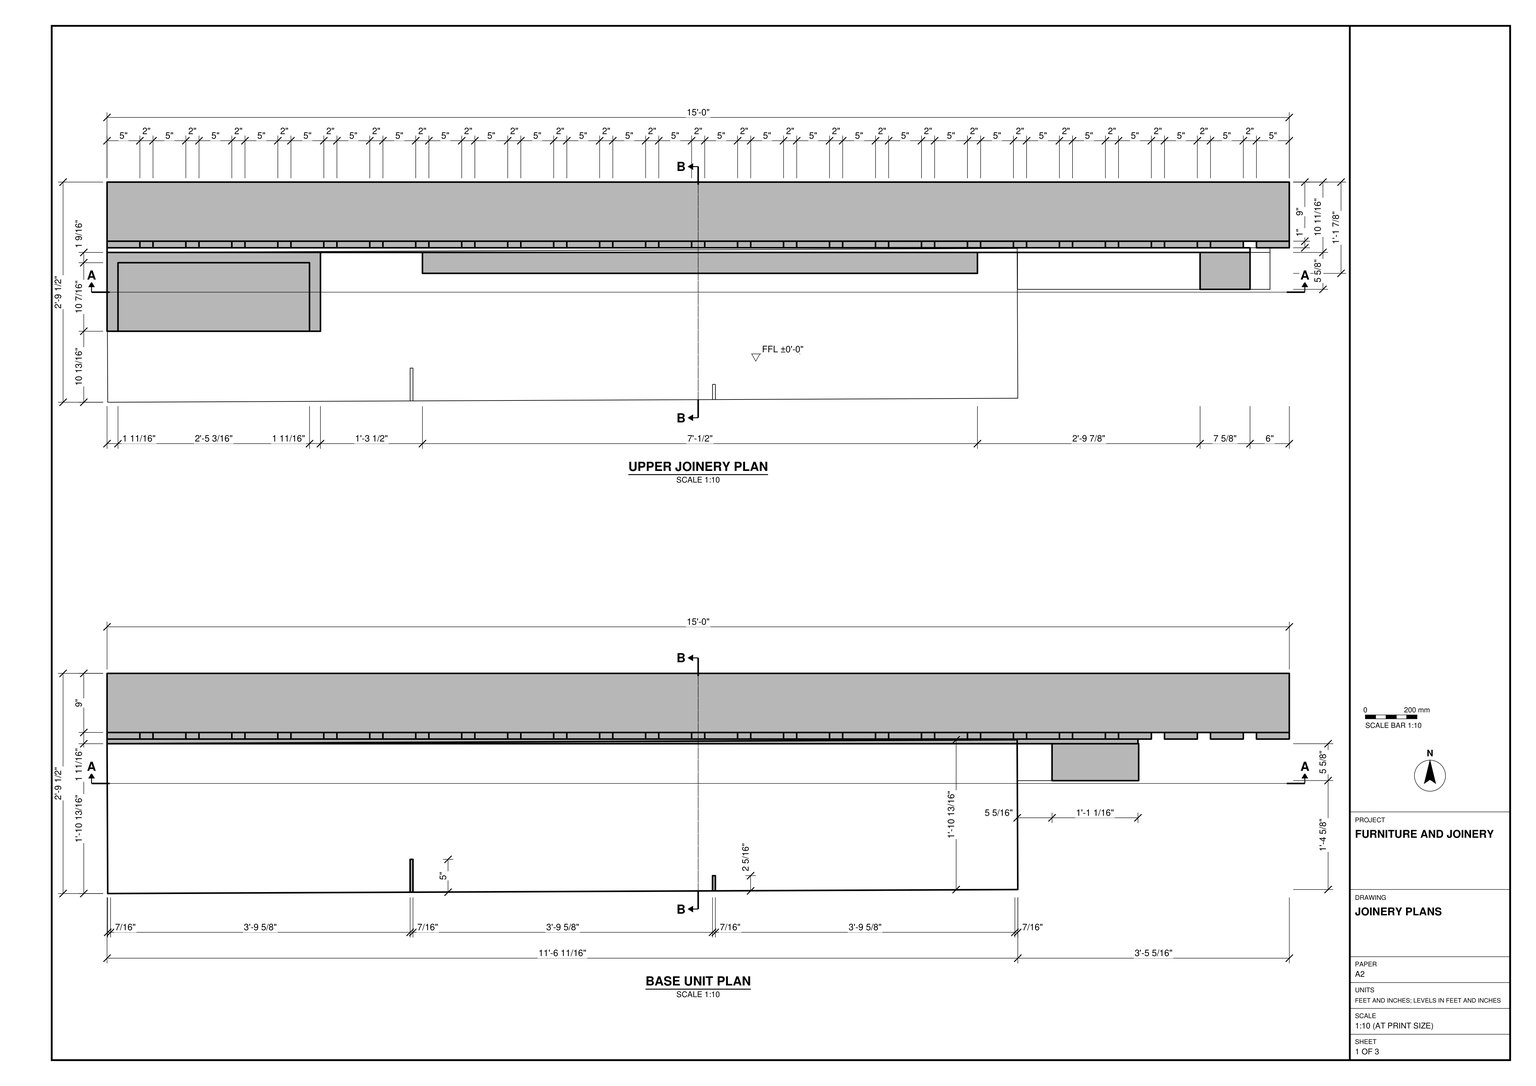
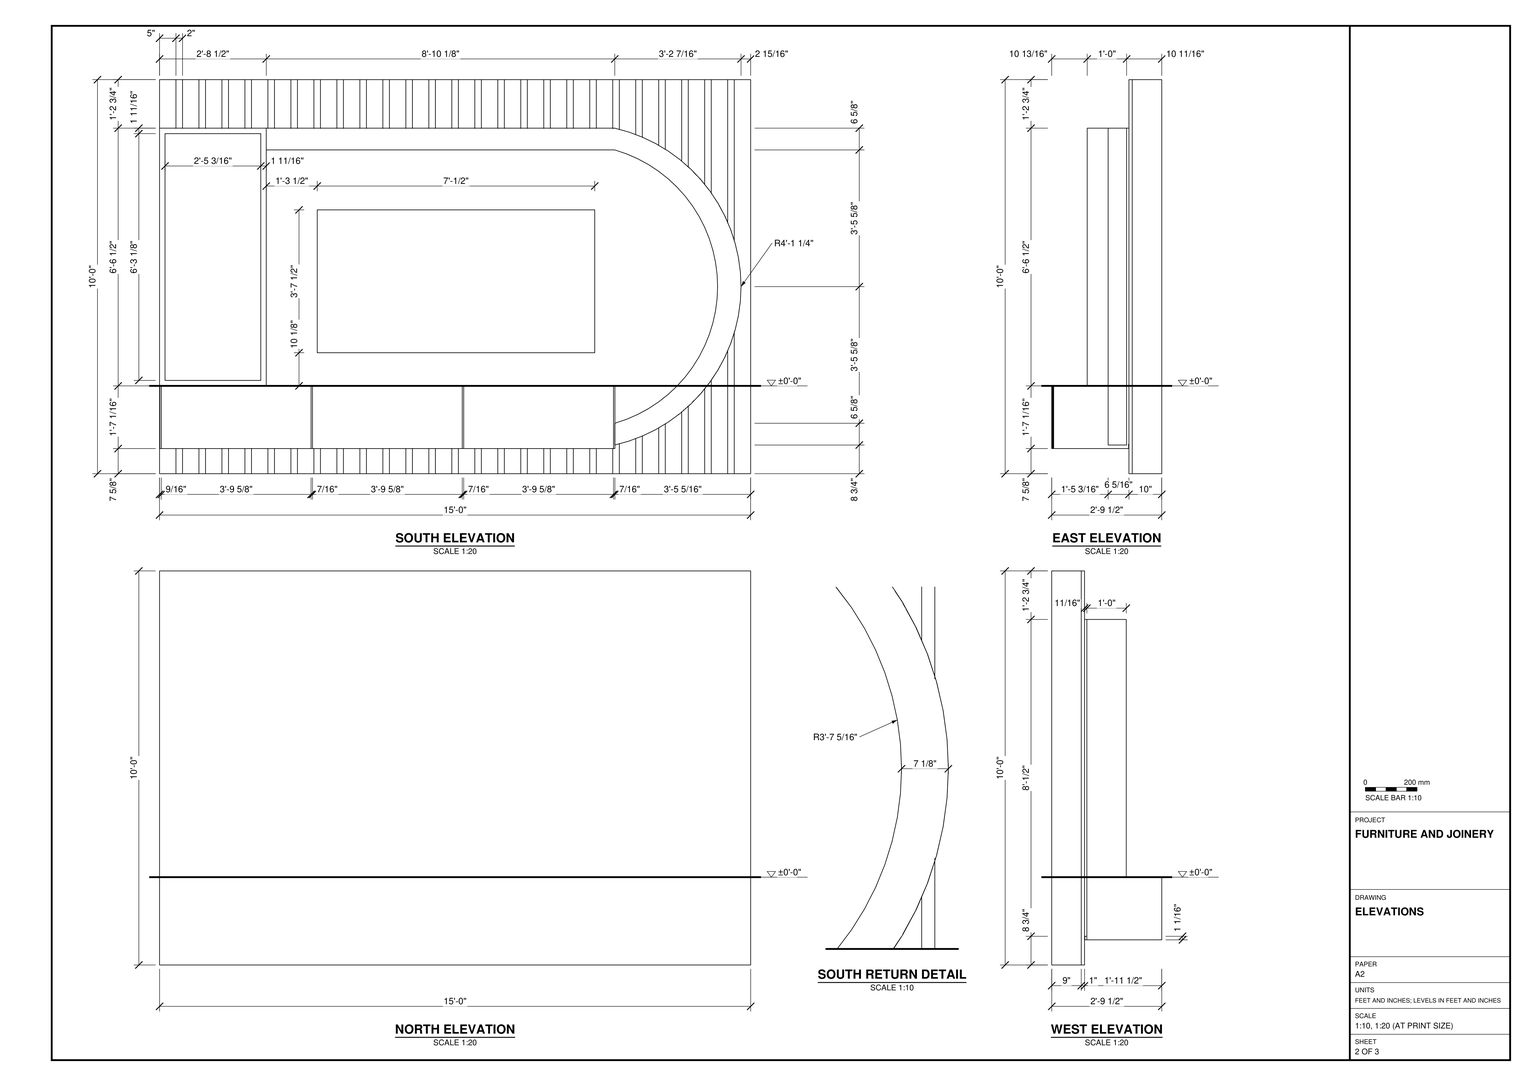
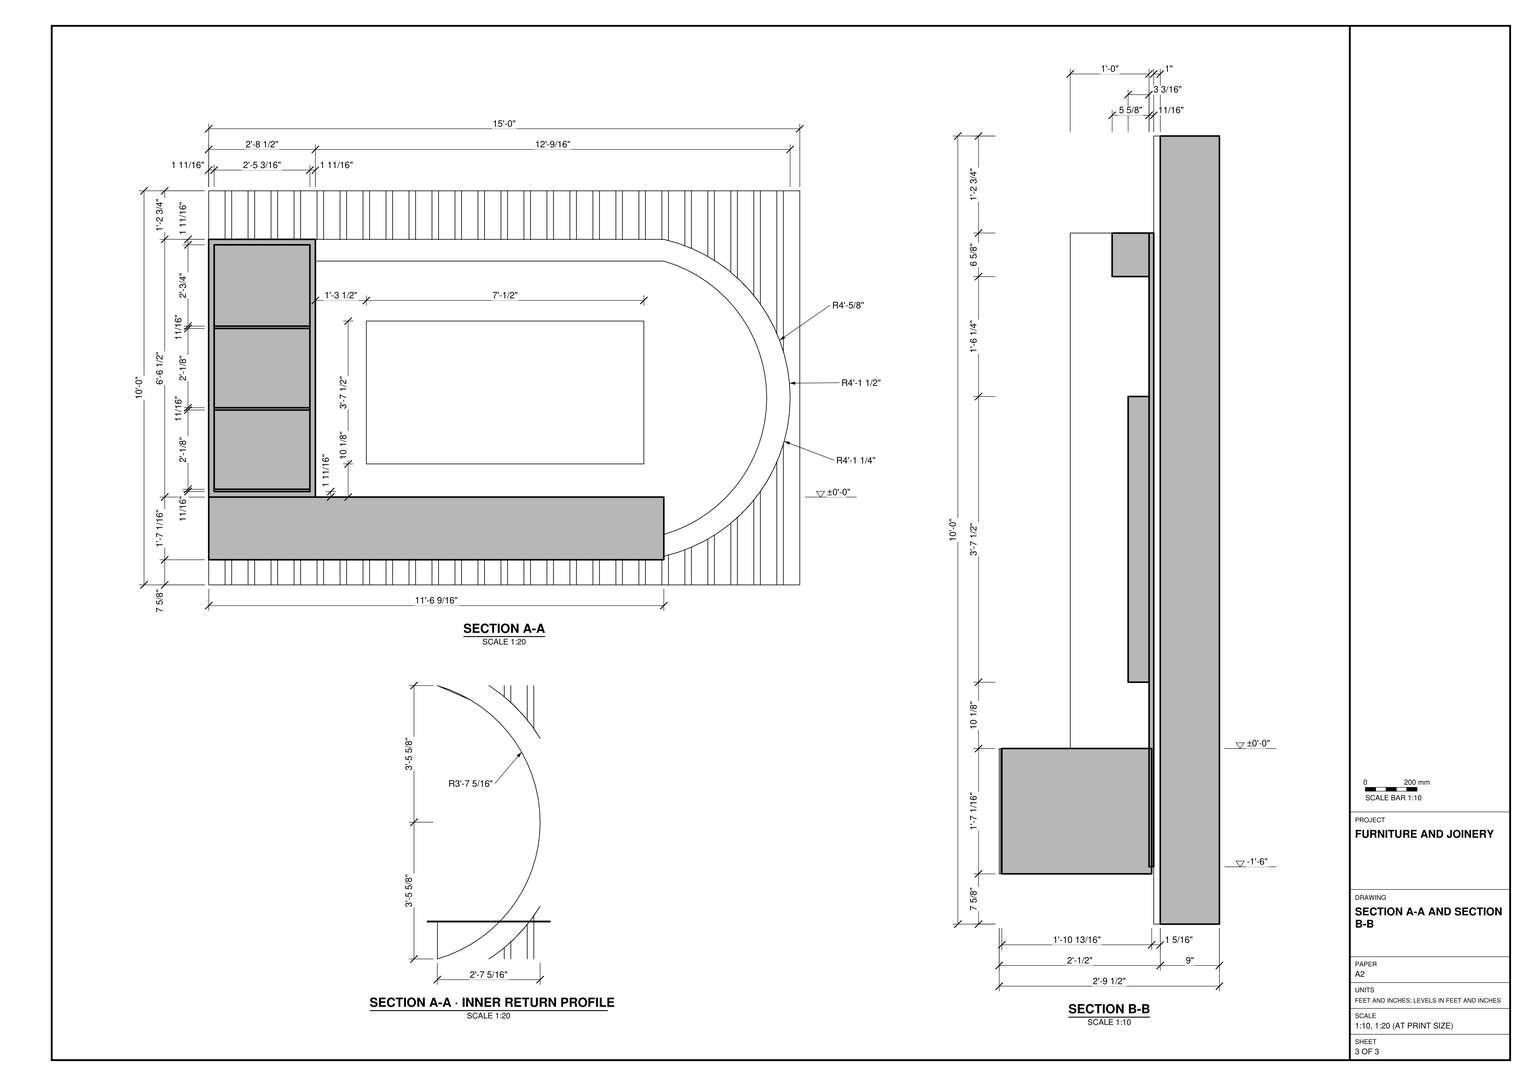
Build the media wall in SketchUp from task_files/diagram_01.pdf. Work in feet and inches. The complete assembly is 15'-0" wide, 2'-9 1/2" deep and 10'-0" high. Use the top of the base unit as the ±0'-0" reference level, not the bottom of the backing.

Start with the rectangular backing. Keep its rear face plain and run vertical slats across its front, leaving the slats visible above, below and to the right of the cabinetry as shown in the south elevation. Project the three-bay base unit forward from the backing. Set the tall shelved cabinet on its left end and place the rectangular screen panel to the right of the cabinet, leaving a gap between the screen and the base top.

Run the upper band horizontally from the tall cabinet, then curve it down around the right side to meet the end of the base. Use the return detail for its inner and outer edges and the plans and sections for the different projections of the cabinet, band, screen and base. Keep distinct joinery pieces in separate groups or components and use components for repeated parts. Any decor or loose items may be suitable library components. Save one SketchUp model as output_files/slatted_media_wall_with_a_curved_return.skp.

# SketchUp Ruby script. Lengths in inches.
U = 1.inch
M = Sketchup.active_model
def pt(a) = Geom::Point3d.new(a.map { |v| v * U })
def face(e, loops, mat)
  f = e.add_face(loops[0].map { |a| pt(a) })
  loops[1..].each { |l| e.add_face(l.map { |a| pt(a) }).erase! }
  f.material = f.back_material = mat if mat
  f
end
# faces: each face lists its corners as indices into pts; further lists are holes
def faces(e, pts, list, mat = nil) = list.each { |f| face(e, (f[0].is_a?(Array) ? f : [f]).map { |l| l.map { |i| pts[i] } }, mat) }
# xy, xz, yz: faces in a plane at the given z, y or x. An outline is a flat list of corners, or four numbers for a rectangle; further outlines are holes
def ring(l) = l.size == 4 ? [[l[0], l[1]], [l[2], l[1]], [l[2], l[3]], [l[0], l[3]]] : l.each_slice(2).to_a
def flat(e, list, mat, &to3) = list.each { |f| face(e, (f[0].is_a?(Array) ? f : [f]).map { |l| ring(l).map { |u, v| to3.(u, v) } }, mat) }
def xy(e, z, list, mat = nil) = flat(e, list, mat) { |x, y| [x, y, z] }
def xz(e, y, list, mat = nil) = flat(e, list, mat) { |x, z| [x, y, z] }
def yz(e, x, list, mat = nil) = flat(e, list, mat) { |y, z| [x, y, z] }
def lines(e, pts, list) = list.each { |a, b| e.add_line(pt(pts[a]), pt(pts[b])) }
# prism: a flat outline (further loops are holes) pulled along v
def prism(e, loops, v, mat = nil)
  f = face(e, loops, mat); d = Geom::Vector3d.new(v.map { |x| x * U })
  f.pushpull(f.normal.samedirection?(d) ? d.length : -d.length)
end
def box(e, o, s, mat = nil) = prism(e, [[o, [o[0] + s[0], o[1], o[2]], [o[0] + s[0], o[1] + s[1], o[2]], [o[0], o[1] + s[1], o[2]]]], [0, 0, s[2]], mat)
def at(x, y, z, deg = 0) = Geom::Transformation.translation(pt([x, y, z])) * Geom::Transformation.rotation(ORIGIN, Z_AXIS, deg.degrees)
def axes(o, x, y, z) = Geom::Transformation.new([*x, 0, *y, 0, *z, 0, *pt(o).to_a, 1])
def part(name) = M.definitions.add(name)
# library, detail: a bought-in or finely detailed component or shape, given as its bounding box
def library(name, o, s) = part(name).tap { |d| box(d.entities, o, s) }
def detail(e, o, s) = box(e.add_group.entities, o, s)
def put(e, d, t, mat = nil) = e.add_instance(d, t).tap { |i| i.material = mat if mat }
def group(e, t, mat = nil) = e.add_group.tap { |g| g.transformation = t; g.material = mat if mat }.entities
root = M.entities
M.materials.add("[Color D01]").color = [255, 242, 204]
M.materials.add("[Color M09]").color = [0, 0, 0]
M.materials.add("[Translucent Glass Gray]").color = [128, 128, 128]
M.materials["[Translucent Glass Gray]"].alpha = 0.5
M.materials.add("[Wood Veneer 01]").color = [120, 70, 37]
c1 = part("Vertical wall slat")
xy(c1.entities,0,[[0,-1,5,0]],"[Wood Veneer 01]")
xy(c1.entities,120,[[0,-1,5,0]],"[Wood Veneer 01]")
xz(c1.entities,-1,[[0,0,5,120]],"[Wood Veneer 01]")
xz(c1.entities,0,[[0,0,5,120]])
yz(c1.entities,0,[[-1,0,0,120]],"[Wood Veneer 01]")
yz(c1.entities,5,[[-1,0,0,120]],"[Wood Veneer 01]")
c2 = part("Group\#11")
box(c2.entities,[0,0,0],[29.16,9.21,0.71])
c3 = part("Group\#8")
xz(c3.entities,0,[[0,0,0.43,19.09]])
put(root,c1,at(175,24.52,0))
put(root,c1,at(168,24.52,0))
put(root,c1,at(161,24.52,0))
put(root,c1,at(154,24.52,0))
put(root,c1,at(147,24.52,0))
put(root,c1,at(140,24.52,0))
put(root,c1,at(133,24.52,0))
put(root,c1,at(126,24.52,0))
put(root,c1,at(119,24.52,0))
put(root,c1,at(112,24.52,0))
put(root,c1,at(105,24.52,0))
put(root,c1,at(98,24.52,0))
put(root,c1,at(91,24.52,0))
put(root,c1,at(84,24.52,0))
put(root,c1,at(77,24.52,0))
put(root,c1,at(70,24.52,0))
put(root,c1,at(63,24.52,0))
put(root,c1,at(56,24.52,0))
put(root,c1,at(49,24.52,0))
put(root,c1,at(42,24.52,0))
put(root,c1,at(35,24.52,0))
put(root,c1,at(28,24.52,0))
put(root,c1,at(21,24.52,0))
put(root,c1,at(14,24.52,0))
put(root,c1,at(7,24.52,0))
put(root,c1,at(0,24.52,0))
g1 = group(root,at(0,24.52,0),"[Color D01]")
box(g1,[0,0,0],[180,9,120])
g2 = group(root,at(0,22.8125,8.73),"[Color D01]")
prism(g2,[[[138,0.71,0],[0,0.71,0],[0,0.71,96.49],[138,0.71,96.49],[142.33,0.71,95.36],[146.54,0.71,93.85],[150.59,0.71,91.96],[154.46,0.71,89.7],[158.11,0.71,87.11],[161.51,0.71,84.2],[164.625,0.71,80.99],[167.44,0.71,77.51],[169.93,0.71,73.8],[172.07,0.71,69.87],[173.85,0.71,65.76],[175.25,0.71,61.51],[176.25,0.71,57.15],[176.86,0.71,52.72],[177.0625,0.71,48.25],[176.86,0.71,43.78],[176.25,0.71,39.34],[175.25,0.71,34.98],[173.85,0.71,30.73],[172.07,0.71,26.625],[169.93,0.71,22.7],[167.44,0.71,18.98],[164.625,0.71,15.5],[161.51,0.71,12.29],[158.11,0.71,9.38],[154.46,0.71,6.79],[150.59,0.71,4.54],[146.54,0.71,2.64],[142.33,0.71,1.13]]],[0,-0.71,0])
g3 = group(root,at(0,22.8125,8.73),"[Color D01]")
xy(g3,18.01,[[0,-12,32.49,0]])
xy(g3,19.68,[[1.67,-12,30.83,-10.78]])
xy(g3,94.82,[[1.67,-12,30.83,-1.5625]])
xy(g3,96.49,[[0,-12,32.49,0]])
xz(g3,-12,[[[0,18.01,32.49,96.49],[1.67,19.68,30.83,94.82]]])
xz(g3,-12,[[1.67,19.68,30.83,94.82]],"[Translucent Glass Gray]")
xz(g3,-1.5625,[[1.67,19.68,30.83,94.82]])
xz(g3,0,[[0,18.01,32.49,96.49]])
yz(g3,0,[[-12,18.01,0,96.49]])
yz(g3,1.67,[[-12,19.68,-1.5625,94.82]])
yz(g3,30.83,[[-12,19.68,-1.5625,94.82]])
yz(g3,32.49,[[-12,18.01,0,96.49]])
put(g3,c2,at(1.67,-10.78,44.51))
put(g3,c2,at(1.67,-10.78,69.35))
put(g3,c2,at(1.67,-10.78,19.68))
g4 = group(root,at(32.49,17.1875,8.73),"[Color D01]")
prism(g4,[[[106.125,5.625,89.87],[0,5.625,89.87],[0,5.625,96.49],[106.125,5.625,96.49],[110.4,5.625,95.31],[114.56,5.625,93.75],[118.55,5.625,91.82],[122.36,5.625,89.54],[125.95,5.625,86.93],[129.29,5.625,84],[132.36,5.625,80.8],[135.125,5.625,77.32],[137.57,5.625,73.62],[139.67,5.625,69.71],[141.42,5.625,65.63],[142.79,5.625,61.41],[143.77,5.625,57.08],[144.37,5.625,52.68],[144.57,5.625,48.25],[144.37,5.625,43.8125],[143.77,5.625,39.41],[142.79,5.625,35.09],[141.42,5.625,30.86],[139.67,5.625,26.78],[137.57,5.625,22.875],[135.125,5.625,19.17],[132.36,5.625,15.7],[129.29,5.625,12.49],[125.95,5.625,9.56],[122.36,5.625,6.95],[118.55,5.625,4.68],[114.56,5.625,2.75],[110.4,5.625,1.18],[106.125,5.625,0],[106.125,5.625,6.625],[109.66,5.625,7.81],[113.07,5.625,9.29],[116.35,5.625,11.07],[119.46,5.625,13.11],[122.38,5.625,15.42],[125.1,5.625,17.97],[127.58,5.625,20.74],[129.82,5.625,23.72],[131.8,5.625,26.875],[133.49,5.625,30.1875],[134.9,5.625,33.64],[136,5.625,37.19],[136.8,5.625,40.83],[137.28,5.625,44.53],[137.4375,5.625,48.25],[137.28,5.625,51.97],[136.8,5.625,55.66],[136,5.625,59.3],[134.9,5.625,62.85],[133.49,5.625,66.3],[131.8,5.625,69.62],[129.82,5.625,72.78],[127.58,5.625,75.75],[125.1,5.625,78.52],[122.38,5.625,81.07],[119.46,5.625,83.38],[116.35,5.625,85.43],[113.07,5.625,87.2],[109.66,5.625,88.68]]],[0,-5.625,0])
p = [[106.125,5.625,0],[0,5.625,0]]
lines(g4,p,[[0,1]])
g5 = group(root,at(0,0,7.65),"[Color D01]")
prism(g5,[[[0,22.8125,0],[138.5625,23.42,0],[138.66,0.61,0],[0.1,0,0]]],[0,0,19.09])
put(root,c3,at(0.1,0,7.65))
g6 = group(root,at(46.14,0.2,7.65))
box(g6,[0,0,0],[0.43,5,19.09])
g7 = group(root,at(92.1875,0.41,7.65))
box(g7,[0,0,0],[0.43,2.3125,19.09])
put(root,c3,at(138.23,0.61,7.65))
g8 = group(root,at(48.02,22.8125,36.83))
xy(g8,0,[[0,-3.1875,84.5,0]],"[Color M09]")
xy(g8,43.5,[[0,-3.1875,84.5,0]],"[Color M09]")
xz(g8,-3.1875,[[0,0,84.5,43.5]],"[Color M09]")
xz(g8,0,[[0,0,84.5,43.5]])
yz(g8,0,[[-3.1875,0,0,43.5]],"[Color M09]")
yz(g8,84.5,[[-3.1875,0,0,43.5]],"[Color M09]")
